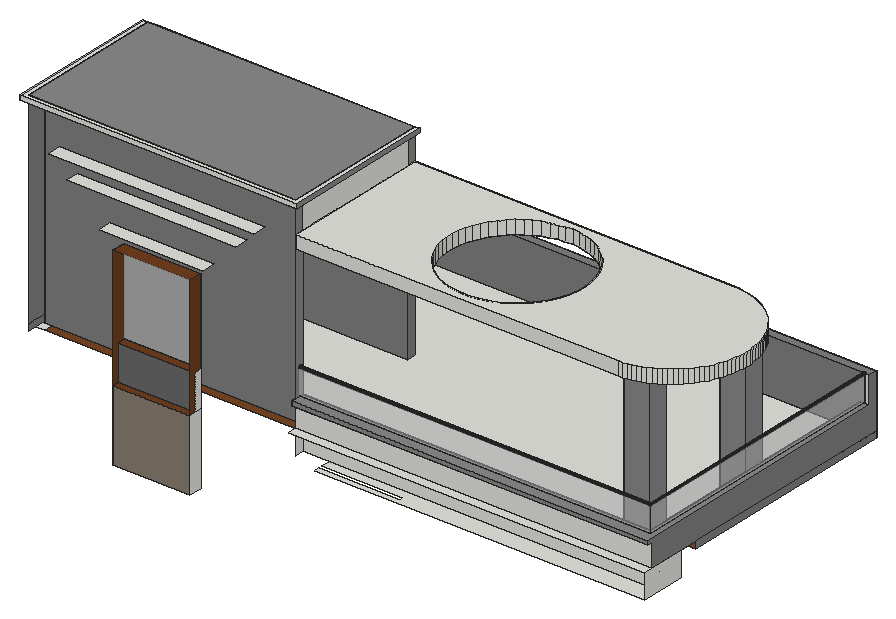
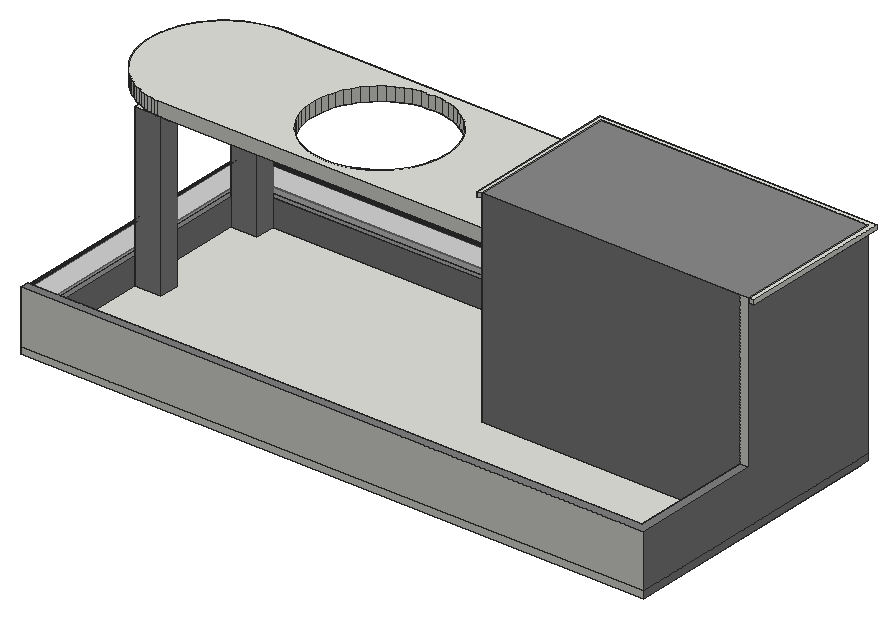
# SketchUp Ruby script. Lengths in inches.
U = 1.inch
M = Sketchup.active_model
def pt(a) = Geom::Point3d.new(a.map { |v| v * U })
def face(e, loops, mat)
  f = e.add_face(loops[0].map { |a| pt(a) })
  loops[1..].each { |l| e.add_face(l.map { |a| pt(a) }).erase! }
  f.material = f.back_material = mat if mat
  f
end
# faces: each face lists its corners as indices into pts; further lists are holes
def faces(e, pts, list, mat = nil) = list.each { |f| face(e, (f[0].is_a?(Array) ? f : [f]).map { |l| l.map { |i| pts[i] } }, mat) }
# xy, xz, yz: faces in a plane at the given z, y or x. An outline is a flat list of corners, or four numbers for a rectangle; further outlines are holes
def ring(l) = l.size == 4 ? [[l[0], l[1]], [l[2], l[1]], [l[2], l[3]], [l[0], l[3]]] : l.each_slice(2).to_a
def flat(e, list, mat, &to3) = list.each { |f| face(e, (f[0].is_a?(Array) ? f : [f]).map { |l| ring(l).map { |u, v| to3.(u, v) } }, mat) }
def xy(e, z, list, mat = nil) = flat(e, list, mat) { |x, y| [x, y, z] }
def xz(e, y, list, mat = nil) = flat(e, list, mat) { |x, z| [x, y, z] }
def yz(e, x, list, mat = nil) = flat(e, list, mat) { |y, z| [x, y, z] }
def lines(e, pts, list) = list.each { |a, b| e.add_line(pt(pts[a]), pt(pts[b])) }
# prism: a flat outline (further loops are holes) pulled along v
def prism(e, loops, v, mat = nil)
  f = face(e, loops, mat); d = Geom::Vector3d.new(v.map { |x| x * U })
  f.pushpull(f.normal.samedirection?(d) ? d.length : -d.length)
end
def box(e, o, s, mat = nil) = prism(e, [[o, [o[0] + s[0], o[1], o[2]], [o[0] + s[0], o[1] + s[1], o[2]], [o[0], o[1] + s[1], o[2]]]], [0, 0, s[2]], mat)
def at(x, y, z, deg = 0) = Geom::Transformation.translation(pt([x, y, z])) * Geom::Transformation.rotation(ORIGIN, Z_AXIS, deg.degrees)
def axes(o, x, y, z) = Geom::Transformation.new([*x, 0, *y, 0, *z, 0, *pt(o).to_a, 1])
def part(name) = M.definitions.add(name)
# library, detail: a bought-in or finely detailed component or shape, given as its bounding box
def library(name, o, s) = part(name).tap { |d| box(d.entities, o, s) }
def detail(e, o, s) = box(e.add_group.entities, o, s)
def put(e, d, t, mat = nil) = e.add_instance(d, t).tap { |i| i.material = mat if mat }
def group(e, t, mat = nil) = e.add_group.tap { |g| g.transformation = t; g.material = mat if mat }.entities
root = M.entities
M.materials.add("[0132_LightGray]").color = [137, 137, 137]
M.materials.add("[0133_Gray]").color = [128, 128, 128]
M.materials.add("[0134_DimGray]").color = [105, 105, 105]
M.materials.add("[Checker Plate]").color = [137, 126, 112]
M.materials.add("[Translucent Glass Gray]1").color = [211, 211, 211]
M.materials["[Translucent Glass Gray]1"].alpha = 0.5
M.materials.add("[Translucent Resin Crush Gray]").color = [184, 184, 184]
M.materials["[Translucent Resin Crush Gray]"].alpha = 0.8
M.materials.add("[Wood Cherry Original]").color = [112, 63, 31]
M.materials.add("[Wood Veneer 01]").color = [120, 70, 37]
xy(root,1012.57,[[268.57,90,475.43,126]],"[Wood Cherry Original]")
xy(root,1182,[[804,102,804,115.125,1021.625,115.125,1021.625,126,804,126,804,150,1666.59,150,1666.59,222,1692,222,1692,102]])
xy(root,1204.57,[[268.57,108,475.43,126]])
xy(root,1204.57,[[268.57,90,475.43,108]],"[Wood Cherry Original]")
xy(root,1230,[[12,150,36,492],[1096.88,313,1090.74,314.24,1085.125,317.03,1080.43,321.18,1076.96,326.4,1074.97,332.34,1074.58,338.59,1075.82,344.73,1078.61,350.34,1082.75,355.04,1087.97,358.5,1093.91,360.5,1100.17,360.89,1106.31,359.65,1111.92,356.86,1116.62,352.71,1120.08,347.49,1122.08,341.55,1122.47,335.3,1121.22,329.16,1118.4375,323.55,1114.29,318.85,1109.07,315.39,1103.13,313.39],[1479.44,313,1473.3,314.24,1467.6875,317.03,1462.99,321.18,1459.53,326.4,1457.53,332.34,1457.14,338.59,1458.38,344.73,1461.17,350.34,1465.32,355.04,1470.54,358.5,1476.48,360.5,1482.73,360.89,1488.87,359.65,1494.48,356.86,1499.18,352.71,1502.64,347.49,1504.64,341.55,1505.03,335.3,1503.79,329.16,1501,323.55,1496.85,318.85,1491.63,315.39,1485.69,313.39],[12,492,36,882],[36,492,1692,882]])
xy(root,1230,[[[36,150,36,492,1692,492,1692,272.8125,1641.1875,272.8125,1641.1875,222,1666.59,222,1666.59,150],[1479.44,313,1485.69,313.39,1491.63,315.39,1496.85,318.85,1501,323.55,1503.79,329.16,1505.03,335.3,1504.64,341.55,1502.64,347.49,1499.18,352.71,1494.48,356.86,1488.87,359.65,1482.73,360.89,1476.48,360.5,1470.54,358.5,1465.32,355.04,1461.17,350.34,1458.38,344.73,1457.14,338.59,1457.53,332.34,1459.53,326.4,1462.99,321.18,1467.6875,317.03,1473.3,314.24],[1096.88,313,1103.13,313.39,1109.07,315.39,1114.29,318.85,1118.4375,323.55,1121.22,329.16,1122.47,335.3,1122.08,341.55,1120.08,347.49,1116.62,352.71,1111.92,356.86,1106.31,359.65,1100.17,360.89,1093.91,360.5,1087.97,358.5,1082.75,355.04,1078.61,350.34,1075.82,344.73,1074.58,338.59,1074.97,332.34,1076.96,326.4,1080.43,321.18,1085.125,317.03,1090.74,314.24]]],"[Wood Veneer 01]")
xy(root,1248,[[732,102,1692,126],[732,126,1692,150],[1668,150,1668,858,36,858,36,528,12,528,12,882,1692,882,1692,150],[36,150,1596,150,1596,204,1668,204,1668,474,1596,474,1596,528,1668,528,1668,858,36,858,36,528,732,528,732,504,36,504],[1596,150,1668,204],
  [1596,474,1668,528]])
xy(root,1300.57,[[268.57,108,475.43,126]],"[Wood Cherry Original]")
xy(root,1308.32,[[732,114,1692,126]],"[0132_LightGray]")
xy(root,1320,[[732,114,1692,114,1692,858,1680,858,1680,138,732,138]],"[0132_LightGray]")
xy(root,1320,[[732,138,1680,138,1680,858,1668,858,1668,150,732,150]],"[0133_Gray]")
xy(root,1392,[[12,528,36,528,36,858,1692,858,1692,882,12,882]],"[0133_Gray]")
xy(root,1531.43,[[268.57,90,475.43,126]],"[Wood Cherry Original]")
xy(root,1567.43,[[232.57,90,511.43,126]])
xy(root,1656,[[144,90,600,126]])
xy(root,1680,[[1596,150,1668,204],[855.78,304.65,849.64,305.89,844.03,308.68,839.33,312.82,835.87,318.04,833.87,323.98,833.48,330.23,834.72,336.375,837.51,341.99,841.66,346.68,846.88,350.15,852.82,352.14,859.07,352.53,865.21,351.29,870.82,348.5,875.52,344.36,878.98,339.14,880.98,333.2,881.37,326.95,880.13,320.8,877.34,315.19,873.19,310.5,867.97,307.03,862.03,305.04],[1497.84,304.65,1491.7,305.89,1486.09,308.68,1481.39,312.82,1477.93,318.04,1475.93,323.98,1475.54,330.23,1476.79,336.375,1479.57,341.99,1483.72,346.68,1488.94,350.15,1494.88,352.14,1501.13,352.53,1507.27,351.29,1512.88,348.5,1517.58,344.36,1521.05,339.14,1523.04,333.2,1523.43,326.95,1522.19,320.8,1519.4,315.19,1515.26,310.5,1510.04,307.03,1504.1,305.04],[1596,474,1596,528,1603.38,528,1613.24,526.95,1624.24,525.15,1635.12,522.75,1645.86,519.75,1656.41,516.16,1666.75,512,1668,511.41,1668,474],[1668,511.41,1668,528,1603.38,528,1613.24,526.95,1624.24,525.15,1635.12,522.75,1645.86,519.75,1656.41,516.16,1666.75,512],
  [1568.75,528,1603.38,528,1602.15,528.13,1591.02,528.7,1579.875,528.66]])
xy(root,1680,[[[732,126,732,528,1596,528,1596,474,1668,474,1668,511.41,1676.84,507.27,1686.66,501.99,1696.17,496.18,1705.35,489.85,1714.16,483.02,1722.58,475.72,1730.59,467.97,1738.15,459.78,1745.25,451.1875,1751.87,442.22,1757.98,432.89,1763.5625,423.25,1768.61,413.31,1773.1,403.1,1777.01,392.67,1780.35,382.03,1783.09,371.23,1785.23,360.29,1786.77,349.25,1787.69,338.14,1788,327,1787.69,315.86,1786.77,304.75,1785.23,293.71,1783.09,282.77,1780.35,271.97,1777.01,261.33,1773.1,250.9,1768.61,240.69,1763.5625,230.75,1757.98,221.11,1751.87,211.78,1745.25,202.8125,1738.15,194.22,1730.59,186.03,1722.58,178.28,1714.16,170.98,1705.35,164.15,1696.17,157.82,1686.66,152.01,1676.84,146.73,1666.75,142,1656.41,137.84,1645.86,134.25,1635.12,131.25,1624.24,128.85,1613.24,127.05,1603.38,126],[1162.36,147.08,1181.2,147.51,1199.89,149.9,1218.22,154.24,1236.01,160.47,1253.04,168.52,1269.14,178.3125,1284.125,189.73,1297.83,202.65,1310.12,216.9375,1320.84,232.43,1329.89,248.95,1337.16,266.34,1342.57,284.38,1346.07,302.9,1347.61,321.67,1347.18,340.51,1344.79,359.2,1340.45,377.53,1334.22,395.32,1326.17,412.35,1316.38,428.45,1304.96,443.43,1292.04,457.14,1277.75,469.43,1262.26,480.15,1245.74,489.2,1228.35,496.47,1210.31,501.88,1191.79,505.38,1173.02,506.92,1154.18,506.49,1135.49,504.1,1117.16,499.76,1099.375,493.53,1082.34,485.48,1066.24,475.6875,1051.26,464.27,1037.55,451.35,1025.26,437.0625,1014.54,421.57,1005.49,405.05,998.22,387.66,992.81,369.62,989.3125,351.1,987.77,332.33,988.2,313.49,990.59,294.8,994.93,276.47,1001.16,258.68,1009.21,241.65,1019,225.55,1030.42,210.57,1043.34,196.86,1057.625,184.57,1073.12,173.85,1089.64,164.8,1107.03,157.53,1125.07,152.12,1143.59,148.62],[855.78,304.65,862.03,305.04,867.97,307.03,873.19,310.5,877.34,315.19,880.13,320.8,881.37,326.95,880.98,333.2,878.98,339.14,875.52,344.36,870.82,348.5,865.21,351.29,859.07,352.53,852.82,352.14,846.88,350.15,841.66,346.68,837.51,341.99,834.72,336.375,833.48,330.23,833.87,323.98,835.87,318.04,839.33,312.82,844.03,308.68,849.64,305.89],[1497.84,304.65,1504.1,305.04,1510.04,307.03,1515.26,310.5,1519.4,315.19,1522.19,320.8,1523.43,326.95,1523.04,333.2,1521.05,339.14,1517.58,344.36,1512.88,348.5,1507.27,351.29,1501.13,352.53,1494.88,352.14,1488.94,350.15,1483.72,346.68,1479.57,341.99,1476.79,336.375,1475.54,330.23,1475.93,323.98,1477.93,318.04,1481.39,312.82,1486.09,308.68,1491.7,305.89]]],"[Wood Veneer 01]")
xy(root,1704,[[96,90,648,126]])
xy(root,1716,[[[732,126,1603.38,126,1613.24,127.05,1624.24,128.85,1635.12,131.25,1645.86,134.25,1656.41,137.84,1666.75,142,1676.84,146.73,1686.66,152.01,1696.17,157.82,1705.35,164.15,1714.16,170.98,1722.58,178.28,1730.59,186.03,1738.15,194.22,1745.25,202.8125,1751.87,211.78,1757.98,221.11,1763.5625,230.75,1768.61,240.69,1773.1,250.9,1777.01,261.33,1780.35,271.97,1783.09,282.77,1785.23,293.71,1786.77,304.75,1787.69,315.86,1788,327,1787.69,338.14,1786.77,349.25,1785.23,360.29,1783.09,371.23,1780.35,382.03,1777.01,392.67,1773.1,403.1,1768.61,413.31,1763.5625,423.25,1757.98,432.89,1751.87,442.22,1745.25,451.1875,1738.15,459.78,1730.59,467.97,1722.58,475.72,1714.16,483.02,1705.35,489.85,1696.17,496.18,1686.66,501.99,1676.84,507.27,1666.75,512,1656.41,516.16,1645.86,519.75,1635.12,522.75,1624.24,525.15,1613.24,526.95,1603.38,528,732,528],[1162.36,147.08,1143.59,148.62,1125.07,152.12,1107.03,157.53,1089.64,164.8,1073.12,173.85,1057.625,184.57,1043.34,196.86,1030.42,210.57,1019,225.55,1009.21,241.65,1001.16,258.68,994.93,276.47,990.59,294.8,988.2,313.49,987.77,332.33,989.3125,351.1,992.81,369.62,998.22,387.66,1005.49,405.05,1014.54,421.57,1025.26,437.0625,1037.55,451.35,1051.26,464.27,1066.24,475.6875,1082.34,485.48,1099.375,493.53,1117.16,499.76,1135.49,504.1,1154.18,506.49,1173.02,506.92,1191.79,505.38,1210.31,501.88,1228.35,496.47,1245.74,489.2,1262.26,480.15,1277.75,469.43,1292.04,457.14,1304.96,443.43,1316.38,428.45,1326.17,412.35,1334.22,395.32,1340.45,377.53,1344.79,359.2,1347.18,340.51,1347.61,321.67,1346.07,302.9,1342.57,284.38,1337.16,266.34,1329.89,248.95,1320.84,232.43,1310.12,216.9375,1297.83,202.65,1284.125,189.73,1269.14,178.3125,1253.04,168.52,1236.01,160.47,1218.22,154.24,1199.89,149.9,1181.2,147.51]]])
xy(root,1776,[[36,150,732,504]])
xy(root,1788,[[0,114,0,528,12,528,12,126,732,126,732,528,744,528,744,114]])
xy(root,1800,[[0,114,744,114,744,528,732,528,732,126,12,126,12,528,0,528]])
xy(root,1800,[[12,126,732,528]],"[0132_LightGray]")
xz(root,90,[[268.57,1012.57,475.43,1204.57]],"[Checker Plate]")
xz(root,108,[[268.57,1204.57,475.43,1300.57]],"[0134_DimGray]")
xz(root,114,[[0,1788,744,1800]])
xz(root,114,[[732,1308.32,1692,1320]],"[0132_LightGray]")
xz(root,126,[[268.57,1012.57,475.43,1204.57],[732,1248,1692,1308.32],[732,1680,1603.38,1716],[12,1788,732,1800]])
xz(root,126,[[268.57,1300.57,475.43,1531.43]],"[Translucent Resin Crush Gray]")
xz(root,138,[[732,1389,1680,1392]])
xz(root,138,[[732,1320,1680,1389]],"[Translucent Glass Gray]1")
xz(root,150,[[732,1182,1666.59,1230],[1596,1248,1668,1320]])
xz(root,150,[[1596,1320,1668,1680]],"[0132_LightGray]")
xz(root,150,[[36,1248,36,1776,732,1776,732,1320,1596,1320,1596,1248]],"[0133_Gray]")
xz(root,204,[[1596,1248,1668,1680]],"[0132_LightGray]")
xz(root,222,[[1666.59,1182,1692,1230]])
xz(root,474,[[1596,1248,1668,1680]],"[0132_LightGray]")
xz(root,504,[[36,1248,732,1776]],"[0133_Gray]")
xz(root,528,[[12,1392,36,1800],[732,1680,1603.38,1716],[0,1788,12,1800],[732,1788,744,1800]])
xz(root,528,[[1596,1248,1668,1680]],"[0132_LightGray]")
xz(root,528,[[36,1248,732,1800]],"[0133_Gray]")
xz(root,858,[[1680,1320,1692,1320,1692,1392,1683,1392,1682.98,1391.6875,1682.93,1391.375,1682.85,1391.07,1682.74,1390.78,1682.6,1390.5,1682.43,1390.24,1682.23,1389.99,1682.01,1389.77,1681.76,1389.57,1681.5,1389.4,1681.22,1389.26,1680.93,1389.15,1680.625,1389.07,1680.3125,1389.02,1680,1389]])
xz(root,858,[[36,1248,1668,1248,1668,1320,1680,1320,1680,1389,1679.6875,1389.02,1679.375,1389.07,1679.07,1389.15,1678.78,1389.26,1678.5,1389.4,1678.24,1389.57,1677.99,1389.77,1677.77,1389.99,1677.57,1390.24,1677.4,1390.5,1677.26,1390.78,1677.15,1391.07,1677.07,1391.375,1677.02,1391.6875,1677,1392,36,1392]],"[0133_Gray]")
xz(root,882,[[12,1230,1692,1248],[12,1248,1692,1392]])
yz(root,0,[[114,1788,528,1800]])
yz(root,12,[[126,1788,528,1800]])
yz(root,12,[[126,1230,882,1248],[126,1248,126,1788,528,1788,528,1392,882,1392,882,1248]],"[0133_Gray]")
yz(root,36,[[150,1248,504,1776],[528,1248,858,1392]],"[0133_Gray]")
yz(root,268.57,[[90,1012.57,126,1204.57],[108,1204.57,126,1300.57]])
yz(root,268.57,[[90,1204.57,108,1204.57,108,1300.57,126,1300.57,126,1531.43,90,1531.43]],"[Wood Cherry Original]")
yz(root,475.43,[[90,1012.57,126,1204.57],[108,1204.57,126,1300.57]])
yz(root,475.43,[[90,1204.57,90,1531.43,126,1531.43,126,1300.57,108,1300.57,108,1204.57]],"[Wood Cherry Original]")
yz(root,732,[[126,1182,150,1230],[114,1308.32,126,1320],[138,1389,137.6875,1389.02,137.375,1389.07,137.07,1389.15,136.78,1389.26,136.5,1389.4,136.24,1389.57,135.99,1389.77,135.77,1389.99,135.57,1390.24,135.4,1390.5,135.26,1390.78,135.15,1391.07,135.07,1391.375,135.02,1391.6875,135,1392,135.02,1392.3125,135.07,1392.625,135.15,1392.93,135.26,1393.22,135.4,1393.5,135.57,1393.76,135.77,1394.01,135.99,1394.23,136.24,1394.43,136.5,1394.6,136.78,1394.74,137.07,1394.85,137.375,1394.93,137.6875,1394.98,138,1395,138.3125,1394.98,138.625,1394.93,138.93,1394.85,139.22,1394.74,139.5,1394.6,139.76,1394.43,140.01,1394.23,140.23,1394.01,140.43,1393.76,140.6,1393.5,140.74,1393.22,140.85,1392.93,140.93,1392.625,140.98,1392.3125,141,1392,140.98,1391.6875,140.93,1391.375,140.85,1391.07,140.74,1390.78,140.6,1390.5,140.43,1390.24,140.23,1389.99,140.01,1389.77,139.76,1389.57,139.5,1389.4,139.22,1389.26,138.93,1389.15,138.625,1389.07,138.3125,1389.02],[126,1680,150,1716],[150,1680,504,1716],
  [504,1680,528,1716],[150,1716,504,1776],[126,1788,528,1800]])
yz(root,732,[[[126,1320,150,1680],[138,1389,137.6875,1389.02,137.375,1389.07,137.07,1389.15,136.78,1389.26,136.5,1389.4,136.24,1389.57,135.99,1389.77,135.77,1389.99,135.57,1390.24,135.4,1390.5,135.26,1390.78,135.15,1391.07,135.07,1391.375,135.02,1391.6875,135,1392,135.02,1392.3125,135.07,1392.625,135.15,1392.93,135.26,1393.22,135.4,1393.5,135.57,1393.76,135.77,1394.01,135.99,1394.23,136.24,1394.43,136.5,1394.6,136.78,1394.74,137.07,1394.85,137.375,1394.93,137.6875,1394.98,138,1395,138.3125,1394.98,138.625,1394.93,138.93,1394.85,139.22,1394.74,139.5,1394.6,139.76,1394.43,140.01,1394.23,140.23,1394.01,140.43,1393.76,140.6,1393.5,140.74,1393.22,140.85,1392.93,140.93,1392.625,140.98,1392.3125,141,1392,140.98,1391.6875,140.93,1391.375,140.85,1391.07,140.74,1390.78,140.6,1390.5,140.43,1390.24,140.23,1389.99,140.01,1389.77,139.76,1389.57,139.5,1389.4,139.22,1389.26,138.93,1389.15,138.625,1389.07,138.3125,1389.02]],[126,1716,150,1776],[504,1716,528,1776],[126,1776,528,1788]],"[0132_LightGray]")
yz(root,732,[[504,1248,528,1680]],"[0133_Gray]")
yz(root,744,[[114,1788,528,1800]],"[0132_LightGray]")
yz(root,1596,[[150,1248,204,1680],[474,1248,528,1680]],"[0132_LightGray]")
yz(root,1666.59,[[150,1182,222,1230]])
yz(root,1668,[[150,1248,204,1320],[474,1248,528,1320]])
yz(root,1668,[[150,1320,204,1680],[474,1320,528,1680]],"[0132_LightGray]")
yz(root,1668,[[204,1248,474,1320],[528,1248,858,1320]],"[0133_Gray]")
yz(root,1680,[[138,1389,858,1392]])
yz(root,1680,[[138,1320,858,1389]],"[Translucent Glass Gray]1")
yz(root,1692,[[102,1182,222,1248]])
yz(root,1692,[[272.8125,1230,882,1248],[126,1248,882,1248,882,1392,858,1392,858,1320,114,1320,114,1308.32,126,1308.32]],"[0133_Gray]")
p = [[732,137.375,1389.07],[732,137.6875,1389.02],[1680.3125,137.6875,1389.02],[1680.625,137.375,1389.07],[1680.3125,858,1389.02],[1680.625,858,1389.07],
  [732,138,1389],[1680,138,1389],[1680,858,1389],[732,138.3125,1389.02],[1679.6875,138.3125,1389.02],[1679.6875,858,1389.02],
  [732,138.625,1389.07],[1679.375,138.625,1389.07],[1679.375,858,1389.07],[732,136.78,1389.26],[732,137.07,1389.15],[1680.93,137.07,1389.15],
  [1681.22,136.78,1389.26],[1680.93,858,1389.15],[1681.22,858,1389.26],[732,138.93,1389.15],[1679.07,138.93,1389.15],[1679.07,858,1389.15],
  [732,139.22,1389.26],[1678.78,139.22,1389.26],[1678.78,858,1389.26],[732,136.5,1389.4],[1681.5,136.5,1389.4],[1681.5,858,1389.4],
  [732,139.5,1389.4],[1678.5,139.5,1389.4],[1678.5,858,1389.4],[732,136.24,1389.57],[1681.76,136.24,1389.57],[1681.76,858,1389.57],
  [732,139.76,1389.57],[1678.24,139.76,1389.57],[1678.24,858,1389.57],[732,135.99,1389.77],[1682.01,135.99,1389.77],[1682.01,858,1389.77],
  [732,140.01,1389.77],[1677.99,140.01,1389.77],[1677.99,858,1389.77],[732,135.77,1389.99],[1682.23,135.77,1389.99],[1682.23,858,1389.99],
  [732,140.23,1389.99],[1677.77,140.23,1389.99],[1677.77,858,1389.99],[732,135.57,1390.24],[1682.43,135.57,1390.24],[1682.43,858,1390.24],
  [732,140.43,1390.24],[1677.57,140.43,1390.24],[1677.57,858,1390.24],[732,135.4,1390.5],[1682.6,135.4,1390.5],[1682.6,858,1390.5],
  [732,140.6,1390.5],[1677.4,140.6,1390.5],[1677.4,858,1390.5],[732,135.26,1390.78],[1682.74,135.26,1390.78],[1682.74,858,1390.78],
  [732,140.74,1390.78],[1677.26,140.74,1390.78],[1677.26,858,1390.78],[732,135.15,1391.07],[1682.85,135.15,1391.07],[1682.85,858,1391.07],
  [732,140.85,1391.07],[1677.15,140.85,1391.07],[1677.15,858,1391.07],[732,135.07,1391.375],[1682.93,135.07,1391.375],[1682.93,858,1391.375],
  [732,140.93,1391.375],[1677.07,140.93,1391.375],[1677.07,858,1391.375],[732,135.02,1391.6875],[1682.98,135.02,1391.6875],[1682.98,858,1391.6875],
  [732,140.98,1391.6875],[1677.02,140.98,1391.6875],[1677.02,858,1391.6875],[732,135,1392],[1683,135,1392],[1683,858,1392],
  [732,141,1392],[1677,141,1392],[1677,858,1392],[732,135.02,1392.3125],[1682.98,135.02,1392.3125],[1682.98,858,1392.3125],
  [732,140.98,1392.3125],[1677.02,140.98,1392.3125],[1677.02,858,1392.3125],[732,135.07,1392.625],[1682.93,135.07,1392.625],[1682.93,858,1392.625],
  [732,140.93,1392.625],[1677.07,140.93,1392.625],[1677.07,858,1392.625],[732,135.15,1392.93],[1682.85,135.15,1392.93],[1682.85,858,1392.93],
  [732,140.85,1392.93],[1677.15,140.85,1392.93],[1677.15,858,1392.93],[732,135.26,1393.22],[1682.74,135.26,1393.22],[1682.74,858,1393.22],
  [732,140.74,1393.22],[1677.26,140.74,1393.22],[1677.26,858,1393.22],[732,135.4,1393.5],[1682.6,135.4,1393.5],[1682.6,858,1393.5],
  [732,140.6,1393.5],[1677.4,140.6,1393.5],[1677.4,858,1393.5],[732,135.57,1393.76],[1682.43,135.57,1393.76],[1682.43,858,1393.76],
  [732,140.43,1393.76],[1677.57,140.43,1393.76],[1677.57,858,1393.76],[732,135.77,1394.01],[1682.23,135.77,1394.01],[1682.23,858,1394.01],
  [732,140.23,1394.01],[1677.77,140.23,1394.01],[1677.77,858,1394.01],[732,135.99,1394.23],[1682.01,135.99,1394.23],[1682.01,858,1394.23],
  [732,140.01,1394.23],[1677.99,140.01,1394.23],[1677.99,858,1394.23],[732,136.24,1394.43],[1681.76,136.24,1394.43],[1681.76,858,1394.43],
  [732,139.76,1394.43],[1678.24,139.76,1394.43],[1678.24,858,1394.43],[732,136.5,1394.6],[1681.5,136.5,1394.6],[1681.5,858,1394.6],
  [732,139.5,1394.6],[1678.5,139.5,1394.6],[1678.5,858,1394.6],[732,136.78,1394.74],[1681.22,136.78,1394.74],[1681.22,858,1394.74],
  [732,139.22,1394.74],[1678.78,139.22,1394.74],[1678.78,858,1394.74],[732,137.07,1394.85],[1680.93,137.07,1394.85],[1680.93,858,1394.85],
  [732,138.93,1394.85],[1679.07,138.93,1394.85],[1679.07,858,1394.85],[732,137.375,1394.93],[1680.625,137.375,1394.93],[1680.625,858,1394.93],
  [732,137.6875,1394.98],[1680.3125,137.6875,1394.98],[1680.3125,858,1394.98],[732,138.625,1394.93],[732,138.3125,1394.98],[1679.6875,138.3125,1394.98],
  [1679.375,138.625,1394.93],[1679.6875,858,1394.98],[1679.375,858,1394.93],[732,138,1395],[1680,138,1395],[1680,858,1395],
  [1603.38,126,1680],[1613.24,127.05,1680],[1613.24,127.05,1716],[1603.38,126,1716],[1624.24,128.85,1680],[1624.24,128.85,1716],
  [1635.12,131.25,1680],[1635.12,131.25,1716],[1645.86,134.25,1680],[1645.86,134.25,1716],[1656.41,137.84,1680],[1656.41,137.84,1716],
  [1666.75,142,1680],[1666.75,142,1716],[1676.84,146.73,1680],[1676.84,146.73,1716],[1686.66,152.01,1680],[1686.66,152.01,1716],
  [1143.59,148.62,1716],[1162.36,147.08,1716],[1162.36,147.08,1680],[1143.59,148.62,1680],[1181.2,147.51,1716],[1181.2,147.51,1680],
  [1199.89,149.9,1716],[1199.89,149.9,1680],[1125.07,152.12,1716],[1125.07,152.12,1680],[1218.22,154.24,1716],[1218.22,154.24,1680],
  [1696.17,157.82,1680],[1696.17,157.82,1716],[1107.03,157.53,1716],[1107.03,157.53,1680],[1236.01,160.47,1716],[1236.01,160.47,1680],
  [1089.64,164.8,1716],[1089.64,164.8,1680],[1705.35,164.15,1680],[1705.35,164.15,1716],[1253.04,168.52,1716],[1253.04,168.52,1680],
  [1714.16,170.98,1680],[1714.16,170.98,1716],[1073.12,173.85,1716],[1073.12,173.85,1680],[1269.14,178.3125,1716],[1269.14,178.3125,1680],
  [1722.58,178.28,1680],[1722.58,178.28,1716],[1057.625,184.57,1716],[1057.625,184.57,1680],[1284.125,189.73,1716],[1284.125,189.73,1680],
  [1730.59,186.03,1680],[1730.59,186.03,1716],[1043.34,196.86,1716],[1043.34,196.86,1680],[1738.15,194.22,1680],[1738.15,194.22,1716],
  [1297.83,202.65,1716],[1297.83,202.65,1680],[1745.25,202.8125,1680],[1745.25,202.8125,1716],[1030.42,210.57,1716],[1030.42,210.57,1680],
  [1310.12,216.9375,1716],[1310.12,216.9375,1680],[1751.87,211.78,1680],[1751.87,211.78,1716],[1019,225.55,1716],[1019,225.55,1680],
  [1757.98,221.11,1680],[1757.98,221.11,1716],[1320.84,232.43,1716],[1320.84,232.43,1680],[1763.5625,230.75,1680],[1763.5625,230.75,1716],
  [1009.21,241.65,1716],[1009.21,241.65,1680],[1768.61,240.69,1680],[1768.61,240.69,1716],[1329.89,248.95,1716],[1329.89,248.95,1680],
  [1773.1,250.9,1680],[1773.1,250.9,1716],[1001.16,258.68,1716],[1001.16,258.68,1680],[1337.16,266.34,1716],[1337.16,266.34,1680],
  [1777.01,261.33,1680],[1777.01,261.33,1716],[994.93,276.47,1716],[994.93,276.47,1680],[1780.35,271.97,1680],[1780.35,271.97,1716],
  [1342.57,284.38,1716],[1342.57,284.38,1680],[1783.09,282.77,1680],[1783.09,282.77,1716],[990.59,294.8,1716],[990.59,294.8,1680],
  [1785.23,293.71,1680],[1785.23,293.71,1716],[1346.07,302.9,1716],[1346.07,302.9,1680],[1786.77,304.75,1680],[1786.77,304.75,1716],
  [988.2,313.49,1716],[988.2,313.49,1680],[1347.61,321.67,1716],[1347.61,321.67,1680],[1787.69,315.86,1680],[1787.69,315.86,1716],
  [987.77,332.33,1716],[987.77,332.33,1680],[1788,327,1680],[1788,327,1716],[1347.18,340.51,1716],[1347.18,340.51,1680],
  [1787.69,338.14,1680],[1787.69,338.14,1716],[989.3125,351.1,1716],[989.3125,351.1,1680],[1786.77,349.25,1680],[1786.77,349.25,1716],
  [1344.79,359.2,1716],[1344.79,359.2,1680],[1785.23,360.29,1680],[1785.23,360.29,1716],[992.81,369.62,1716],[992.81,369.62,1680],
  [1340.45,377.53,1716],[1340.45,377.53,1680],[1783.09,371.23,1680],[1783.09,371.23,1716],[998.22,387.66,1716],[998.22,387.66,1680],
  [1780.35,382.03,1680],[1780.35,382.03,1716],[1334.22,395.32,1716],[1334.22,395.32,1680],[1777.01,392.67,1680],[1777.01,392.67,1716],
  [1005.49,405.05,1716],[1005.49,405.05,1680],[1773.1,403.1,1680],[1773.1,403.1,1716],[1326.17,412.35,1716],[1326.17,412.35,1680],
  [1768.61,413.31,1680],[1768.61,413.31,1716],[1014.54,421.57,1716],[1014.54,421.57,1680],[1316.38,428.45,1716],[1316.38,428.45,1680],
  [1763.5625,423.25,1680],[1763.5625,423.25,1716],[1025.26,437.0625,1716],[1025.26,437.0625,1680],[1757.98,432.89,1680],[1757.98,432.89,1716],
  [1304.96,443.43,1716],[1304.96,443.43,1680],[1751.87,442.22,1680],[1751.87,442.22,1716],[1037.55,451.35,1716],[1037.55,451.35,1680],
  [1745.25,451.1875,1680],[1745.25,451.1875,1716],[1292.04,457.14,1716],[1292.04,457.14,1680],[1738.15,459.78,1680],[1738.15,459.78,1716],
  [1051.26,464.27,1716],[1051.26,464.27,1680],[1277.75,469.43,1716],[1277.75,469.43,1680],[1730.59,467.97,1680],[1730.59,467.97,1716],
  [1066.24,475.6875,1716],[1066.24,475.6875,1680],[1722.58,475.72,1680],[1722.58,475.72,1716],[1262.26,480.15,1716],[1262.26,480.15,1680],
  [1082.34,485.48,1716],[1082.34,485.48,1680],[1714.16,483.02,1680],[1714.16,483.02,1716],[1245.74,489.2,1716],[1245.74,489.2,1680],
  [1705.35,489.85,1680],[1705.35,489.85,1716],[1099.375,493.53,1716],[1099.375,493.53,1680],[1228.35,496.47,1716],[1228.35,496.47,1680],
  [1696.17,496.18,1680],[1696.17,496.18,1716],[1117.16,499.76,1716],[1117.16,499.76,1680],[1686.66,501.99,1680],[1686.66,501.99,1716],
  [1210.31,501.88,1716],[1210.31,501.88,1680],[1135.49,504.1,1716],[1135.49,504.1,1680],[1191.79,505.38,1716],[1191.79,505.38,1680],
  [1676.84,507.27,1680],[1676.84,507.27,1716],[1154.18,506.49,1716],[1154.18,506.49,1680],[1173.02,506.92,1716],[1173.02,506.92,1680],
  [1668,511.41,1680],[1666.75,512,1680],[1666.75,512,1716],[1656.41,516.16,1680],[1656.41,516.16,1716],[1645.86,519.75,1680],
  [1645.86,519.75,1716],[1635.12,522.75,1680],[1635.12,522.75,1716],[1624.24,525.15,1680],[1624.24,525.15,1716],[1613.24,526.95,1680],
  [1613.24,526.95,1716],[1603.38,528,1680],[1603.38,528,1716],[1666.59,150,1230],[1692,150,1230]]
faces(root,p,[[0,1,2,3],[1,6,7,2],[6,9,10,7],[9,12,13,10],[15,16,17,18],[16,0,3,17],[12,21,22,13],[21,24,25,22],
  [27,15,18,28],[24,30,31,25],[33,27,28,34],[30,36,37,31],[39,33,34,40],[36,42,43,37],[45,39,40,46],[42,48,49,43],
  [51,45,46,52],[48,54,55,49],[57,51,52,58],[54,60,61,55],[63,57,58,64],[60,66,67,61],[69,63,64,70],[66,72,73,67],
  [75,69,70,76],[72,78,79,73],[81,75,76,82],[78,84,85,79],[87,81,82,88],[84,90,91,85],[93,87,88,94],[90,96,97,91],
  [99,93,94,100],[96,102,103,97],[105,99,100,106],[102,108,109,103],[111,105,106,112],[108,114,115,109],[117,111,112,118],[114,120,121,115],
  [123,117,118,124],[120,126,127,121],[129,123,124,130],[126,132,133,127],[135,129,130,136],[132,138,139,133],[141,135,136,142],[138,144,145,139],
  [147,141,142,148],[144,150,151,145],[153,147,148,154],[150,156,157,151],[159,153,154,160],[156,162,163,157],[165,159,160,166],[168,165,166,169],
  [171,172,173,174],[162,171,174,163],[177,168,169,178],[172,177,178,173]],"[0133_Gray]")
faces(root,p,[[3,2,4,5],[2,7,8,4],[7,10,11,8],[10,13,14,11],[18,17,19,20],[17,3,5,19],[13,22,23,14],[22,25,26,23],
  [28,18,20,29],[25,31,32,26],[34,28,29,35],[31,37,38,32],[40,34,35,41],[37,43,44,38],[46,40,41,47],[43,49,50,44],
  [52,46,47,53],[49,55,56,50],[58,52,53,59],[55,61,62,56],[64,58,59,65],[61,67,68,62],[70,64,65,71],[67,73,74,68],
  [76,70,71,77],[73,79,80,74],[82,76,77,83],[79,85,86,80],[88,82,83,89],[85,91,92,86],[94,88,89,95],[91,97,98,92],
  [100,94,95,101],[97,103,104,98],[106,100,101,107],[103,109,110,104],[112,106,107,113],[109,115,116,110],[118,112,113,119],[115,121,122,116],
  [124,118,119,125],[121,127,128,122],[130,124,125,131],[127,133,134,128],[136,130,131,137],[133,139,140,134],[142,136,137,143],[139,145,146,140],
  [148,142,143,149],[145,151,152,146],[154,148,149,155],[151,157,158,152],[160,154,155,161],[157,163,164,158],[166,160,161,167],[169,166,167,170],
  [174,173,175,176],[163,174,176,164],[178,169,170,179],[173,178,179,175]],"[0134_DimGray]")
faces(root,p,[[180,181,182,183],[181,184,185,182],[184,186,187,185],[186,188,189,187],[188,190,191,189],[190,192,193,191],[192,194,195,193],[194,196,197,195],
  [198,199,200,201],[199,202,203,200],[202,204,205,203],[206,198,201,207],[204,208,209,205],[196,210,211,197],[212,206,207,213],[208,214,215,209],
  [216,212,213,217],[210,218,219,211],[214,220,221,215],[218,222,223,219],[224,216,217,225],[220,226,227,221],[222,228,229,223],[230,224,225,231],
  [226,232,233,227],[228,234,235,229],[236,230,231,237],[234,238,239,235],[232,240,241,233],[238,242,243,239],[244,236,237,245],[240,246,247,241],
  [242,248,249,243],[250,244,245,251],[248,252,253,249],[246,254,255,247],[252,256,257,253],[258,250,251,259],[256,260,261,257],[254,262,263,255],
  [260,264,265,261],[266,258,259,267],[262,268,269,263],[264,270,271,265],[272,266,267,273],[270,274,275,271],[268,276,277,269],[274,278,279,275],
  [280,272,273,281],[278,282,283,279],[276,284,285,277],[282,286,287,283],[288,280,281,289],[284,290,291,285],[286,292,293,287],[294,288,289,295],
  [292,296,297,293],[290,298,299,291],[296,300,301,297],[302,294,295,303],[300,304,305,301],[298,306,307,299],[304,308,309,305],[310,302,303,311],
  [306,312,313,307],[308,314,315,309],[316,310,311,317],[314,318,319,315],[312,320,321,313],[318,322,323,319],[324,316,317,325],[322,326,327,323],
  [320,328,329,321],[326,330,331,327],[332,324,325,333],[328,334,335,329],[330,336,337,331],[338,332,333,339],[336,340,341,337],[334,342,343,335],
  [340,344,345,341],[346,338,339,347],[344,348,349,345],[342,350,351,343],[348,352,353,349],[354,346,347,355],[350,356,357,351],[352,358,359,353],
  [360,354,355,361],[358,362,363,359],[356,364,365,357],[366,360,361,367],[362,368,369,363],[364,370,371,365],[368,372,373,369],[374,366,367,375],
  [370,376,377,371],[372,378,379,373],[380,374,375,381],[378,382,383,379],[376,384,385,377],[386,380,381,387],[384,388,389,385],[382,390,391,383],
  [392,386,387,393],[388,394,395,389],[394,392,393,395],[396,397,398,391,390],[397,399,400,398],[399,401,402,400],[401,403,404,402],[403,405,406,404],
  [405,407,408,406],[407,409,410,408]])
lines(root,p,[[411,412]])
